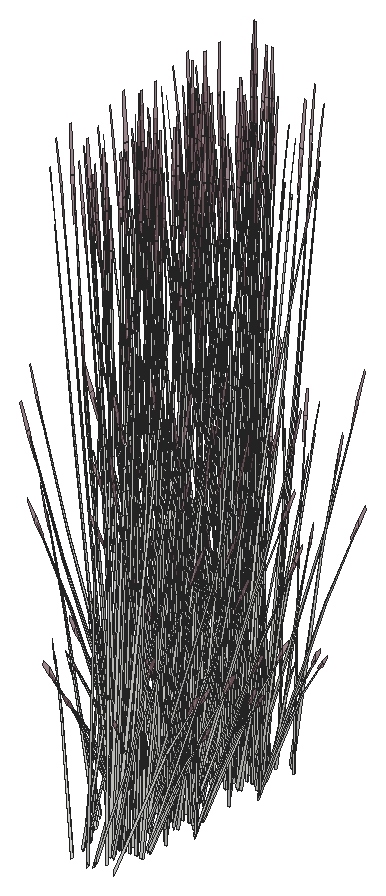
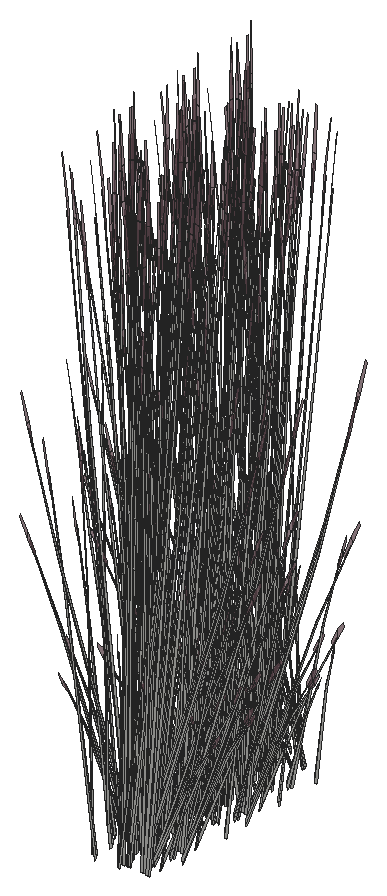
# SketchUp Ruby script. Lengths in inches.
U = 1.inch
M = Sketchup.active_model
def pt(a) = Geom::Point3d.new(a.map { |v| v * U })
def face(e, loops, mat)
  f = e.add_face(loops[0].map { |a| pt(a) })
  loops[1..].each { |l| e.add_face(l.map { |a| pt(a) }).erase! }
  f.material = f.back_material = mat if mat
  f
end
# faces: each face lists its corners as indices into pts; further lists are holes
def faces(e, pts, list, mat = nil) = list.each { |f| face(e, (f[0].is_a?(Array) ? f : [f]).map { |l| l.map { |i| pts[i] } }, mat) }
# xy, xz, yz: faces in a plane at the given z, y or x. An outline is a flat list of corners, or four numbers for a rectangle; further outlines are holes
def ring(l) = l.size == 4 ? [[l[0], l[1]], [l[2], l[1]], [l[2], l[3]], [l[0], l[3]]] : l.each_slice(2).to_a
def flat(e, list, mat, &to3) = list.each { |f| face(e, (f[0].is_a?(Array) ? f : [f]).map { |l| ring(l).map { |u, v| to3.(u, v) } }, mat) }
def xy(e, z, list, mat = nil) = flat(e, list, mat) { |x, y| [x, y, z] }
def xz(e, y, list, mat = nil) = flat(e, list, mat) { |x, z| [x, y, z] }
def yz(e, x, list, mat = nil) = flat(e, list, mat) { |y, z| [x, y, z] }
def lines(e, pts, list) = list.each { |a, b| e.add_line(pt(pts[a]), pt(pts[b])) }
# prism: a flat outline (further loops are holes) pulled along v
def prism(e, loops, v, mat = nil)
  f = face(e, loops, mat); d = Geom::Vector3d.new(v.map { |x| x * U })
  f.pushpull(f.normal.samedirection?(d) ? d.length : -d.length)
end
def box(e, o, s, mat = nil) = prism(e, [[o, [o[0] + s[0], o[1], o[2]], [o[0] + s[0], o[1] + s[1], o[2]], [o[0], o[1] + s[1], o[2]]]], [0, 0, s[2]], mat)
def at(x, y, z, deg = 0) = Geom::Transformation.translation(pt([x, y, z])) * Geom::Transformation.rotation(ORIGIN, Z_AXIS, deg.degrees)
def axes(o, x, y, z) = Geom::Transformation.new([*x, 0, *y, 0, *z, 0, *pt(o).to_a, 1])
def part(name) = M.definitions.add(name)
# library, detail: a bought-in or finely detailed component or shape, given as its bounding box
def library(name, o, s) = part(name).tap { |d| box(d.entities, o, s) }
def detail(e, o, s) = box(e.add_group.entities, o, s)
def put(e, d, t, mat = nil) = e.add_instance(d, t).tap { |i| i.material = mat if mat }
def group(e, t, mat = nil) = e.add_group.tap { |g| g.transformation = t; g.material = mat if mat }.entities
root = M.entities
M.materials.add("LightPink_Translucent").color = [144, 107, 117]
M.materials["LightPink_Translucent"].alpha = 0.75
c1 = part("blade")
p = [[2.15,0.21,22],[0,0.17,0],[0.09,0.45,0],[2.18,0.31,22],[2.29,0.31,22],[0.38,0.45,0],
  [2.48,0.24,33],[2.49,0.24,33],[2.48,0.22,33]]
faces(c1.entities,p,[[0,1,2,3],[4,5,2,3],[6,3,4,7],[8,0,3,6]])
c2 = part("seeds")
p = [[0.3,-0.1,1.38],[-0.01,-0.03,1.59],[-0.01,-0.03,0.03],[0.14,-0.07,-0.07],[0.29,-0.03,3],[0.15,0.01,3.11]]
faces(c2.entities,p,[[0,1,2,3],[1,0,4,5]],"LightPink_Translucent")
c3 = part("blade with seeds")
put(c3.entities,c1,at(0,0,0))
put(c3.entities,c2,axes([2.4,0.25,30.99],[1.5799,-0.05474,1.17369],[-0.12525,1.92788,0.29478],[-0.07173,-0.02425,1.56792]))
put(root,c3,axes([428.55,445.8,152.09],[0.44036,-0.12519,0.14904],[0.10874,0.46588,0.29641],[-0.03927,-0.06788,1.35512]))
put(root,c3,axes([429.46,444.04,152.25],[0.41376,-0.31314,-0.2458],[0.27514,0.44246,-0.42242],[0.10209,0.04493,1.34921]))
put(root,c3,axes([430.08,442.71,152],[0.25622,0.47263,0],[-0.42866,0.26357,-0.43598],[-0.09763,0.06003,1.38303]))
put(root,c3,axes([430.17,448.55,154.21],[0.01066,-0.43628,-0.60019],[0.44902,0.0293,0.07243],[0.04739,-0.18483,0.84903]))
put(root,c3,axes([430.48,442.87,151.26],[0.02986,-0.06809,1.48974],[0.37589,-0.20055,-0.22758],[0.11396,0.1038,0.25375]))
put(root,c3,axes([429.86,440.84,152.4],[-0.01119,-0.44408,1.19347],[0.50665,0.11511,0.50532],[-0.11983,0.243,1.12654]))
put(root,c3,axes([429.78,444.55,151.86],[0.45849,0,0],[0,0.4883,0],[0,0,1.50718]))
put(root,c3,axes([427.03,442.82,151.26],[0.05497,0.04712,1.48974],[0.09321,0.43661,-0.22758],[-0.12183,0.0931,0.25375]))
put(root,c3,axes([429,445.17,152.25],[-0.41376,0.31314,-0.2458],[-0.27514,-0.44246,-0.42242],[-0.10209,-0.04493,1.34921]))
put(root,c3,axes([429.91,443.41,152.09],[-0.44036,0.12519,0.14904],[-0.10874,-0.46588,0.29641],[0.03927,0.06788,1.35512]))
put(root,c3,axes([429.46,447.09,152.34],[0.05257,0.27504,0.97034],[-0.29163,-0.15233,0.71294],[0.03138,-0.14083,0.21373]))
put(root,c3,axes([430.46,442.99,152.25],[-0.26279,-0.01479,0.88755],[0.17355,-0.31417,0.49003],[0.10382,0.11162,0.6962]))
put(root,c3,axes([429.63,444.31,152.01],[-0.51796,-0.09937,0.41563],[0.10541,-0.56124,0.1631],[0.07569,0.05419,1.44303]))
put(root,c3,axes([429.21,445.69,151.86],[-0.13371,-0.40664,0],[0.38182,-0.1424,0],[0,0,1.30413]))
put(root,c3,axes([428.96,445.31,152.21],[-0.07906,0.42093,0.12232],[-0.38625,-0.07307,-0.3493],[-0.07029,-0.04322,1.07074]))
put(root,c3,axes([429.71,445.63,151.85],[0.43024,-0.16003,-0.16218],[0.15118,0.46099,0.00007],[0.04749,-0.01769,1.46908]))
put(root,c3,axes([429.86,445.83,152.09],[0.11838,-0.46875,0.14904],[0.43321,0.13265,0.29641],[-0.07483,0.00228,1.35512]))
put(root,c3,axes([429.77,444.76,151.87],[0.28606,0.30466,0],[-0.28606,0.30466,0],[0,0,1.42996]))
put(root,c3,axes([430.54,444.63,152.09],[-0.32198,-0.34356,0.14904],[0.32447,-0.33323,0.29641],[-0.03556,0.07016,1.35512]))
put(root,c3,axes([429.6,442.22,152.1875],[0.00723,-0.15635,1.20808],[0.34559,-0.17464,-0.25981],[0.10668,0.18713,0.51652]))
put(root,c3,axes([427.96,447.42,152.34],[0.21377,0.16416,0.97034],[-0.31132,0.09868,0.71294],[-0.06661,-0.12616,0.21373]))
put(root,c3,axes([431.83,444.95,152.34],[-0.2532,0.07787,0.97034],[0.11918,-0.32181,0.71294],[0.13432,0.02202,0.21373]))
put(root,c3,axes([428.47,448.29,154.21],[-0.34944,-0.22798,-0.60019],[0.24834,-0.39949,0.07243],[-0.1266,-0.13612,0.84903]))
put(root,c3,axes([429.12,445.875,151.86],[-0.41314,-0.21175,0],[0.19883,-0.43999,0],[0,0,1.37455]))
put(root,c3,axes([429.46,445.3125,152.08],[-0.40016,-0.37963,-0.21282],[0.33672,-0.42629,0.46574],[-0.10776,0.04441,1.42109]))
put(root,c3,axes([428.41,446.04,152.09],[0.38354,0.23583,0.41945],[-0.22925,0.42288,0],[-0.08735,-0.05371,1.33059]))
put(root,c3,axes([428.03,443.53,152.34],[-0.01061,-0.28045,0.97034],[0.26501,0.20003,0.71294],[-0.05212,0.13367,0.21373]))
put(root,c3,axes([429.76,444.41,152.3],[0.19883,-0.425,0.37796],[0.41314,0.20454,-0.1819],[0,0.09797,1.2135]))
put(root,c3,axes([428.73,442.86,151.26],[0.06632,-0.02567,1.48974],[0.39894,0.14126,-0.22758],[0.01167,0.15921,0.25375]))
put(root,c3,axes([429.68,444.65,151.9375],[0,0.54548,-0.04762],[-0.51243,0,0],[0,0.01714,1.5153]))
put(root,c3,axes([427.79,447.91,151.26],[-0.0397,0.06213,1.48974],[-0.40116,0.13396,-0.22758],[-0.09691,-0.12186,0.25375]))
put(root,c3,axes([428.1875,446.29,152],[-0.25622,0.47263,0],[-0.42866,-0.26357,-0.43598],[-0.09763,-0.06003,1.38303]))
put(root,c3,axes([430.8,444.64,152.09],[0,-0.47166,0.41945],[0.45849,0,0],[0,0.10742,1.33059]))
put(root,c3,axes([429.66,445,152.3],[0.44501,-0.02912,0.37796],[0.04024,0.48332,-0.1819],[-0.07967,0.04899,1.2135]))
put(root,c3,axes([429.93,444.5,152.21],[0.38182,-0.13755,0.12232],[0.13371,0.39278,-0.3493],[0,0.08644,1.07074]))
put(root,c3,axes([427.8125,442.92,152.38],[0.37228,-0.08352,0.05498],[0.08559,0.3365,-0.7291],[-0.0236,0.17034,0.65354]))
put(root,c3,axes([430.7,448.14,151.26],[-0.06134,-0.03716,1.48974],[-0.15755,-0.41512,-0.22758],[0.10629,-0.11265,0.25375]))
put(root,c3,axes([431.35,445.46,152.1875],[-0.0987,-0.116,1.20808],[0.12841,-0.38374,-0.25981],[0.19968,0.05198,0.51652]))
put(root,c3,axes([429.59,445.88,151.86],[0.41314,0.21175,0],[-0.19883,0.43999,0],[0,0,1.47801]))
put(root,c3,axes([430.7,449.3125,154.21],[0.21406,-0.37215,-0.60019],[0.37511,0.26448,0.07243],[0.12781,-0.13483,0.84903]))
put(root,c3,axes([428.38,448.23,152],[-0.25622,-0.47263,0],[0.42866,-0.26357,-0.43598],[0.09763,-0.06003,1.38303]))
put(root,c3,axes([429.75,446.35,151.85],[-0.25302,-0.47428,-0.04344],[0.42866,-0.26357,0.43598],[-0.10563,0.04516,1.38235]))
put(root,c3,axes([429.66,445.2,152.21],[0.30276,0.28338,0.12232],[-0.25254,0.31972,-0.3493],[-0.07029,0.04322,1.07074]))
put(root,c3,axes([428.95,447.66,151.8],[-0.28319,0.27058,-0.03288],[-0.25948,-0.29635,-0.1491],[-0.01827,-0.08397,0.4918]))
put(root,c3,axes([428.85,442.68,154.21],[0.19559,0.38351,-0.60019],[-0.40262,0.21373,0.07243],[0.04574,0.1853,0.84903]))
put(root,c3,axes([430.45,445.69,154.21],[0.40965,0.01136,-0.60019],[-0.02751,0.47821,0.07243],[0.17355,0.05047,0.84903]))
put(root,c3,axes([427.72,443.28,152.1875],[0.12932,-0.07441,1.20808],[0.31929,0.22435,-0.25981],[-0.09503,0.19413,0.51652]))
put(root,c3,axes([429.99,446.08,152.09],[0.38354,-0.23583,0.41945],[0.22925,0.42288,0],[-0.08735,0.05371,1.33059]))
put(root,c3,axes([429.44,445.71,151.9375],[0.17817,0.54185,-0.05079],[-0.50909,0.18987,0],[0.00622,0.01892,1.45452]))
put(root,c3,axes([426.88,445.46,152.1875],[0.14242,0.03872,1.20808],[0.09179,0.39548,-0.25981],[-0.19345,0.07403,0.51652]))
put(root,c3,axes([431.01,448.97,152.1875],[-0.1464,-0.01397,1.20808],[-0.14998,-0.37477,-0.25981],[0.17985,-0.10602,0.51652]))
put(root,c3,axes([431.12,444.72,152.01],[0.51243,0,0],[0,0.52715,-0.43598],[0,0.12006,1.38303]))
put(root,c3,axes([430.91,445,151.86],[-0.51218,-0.00377,-0.04204],[0,-0.52715,0.42192],[-0.0161,0.12,1.33776]))
put(root,c3,axes([429.8,444.54,152.25],[0.46151,0.22505,-0.2458],[-0.22222,0.475,-0.42242],[0.0145,0.11662,1.34921]))
put(root,c3,axes([431.18,448.28,152.34],[-0.1365,0.2401,0.97034],[-0.11733,-0.32258,0.71294],[0.11274,-0.08083,0.21373]))
put(root,c3,axes([426.58,446.29,152.34],[0.17079,-0.21377,0.97034],[0.06739,0.33841,0.71294],[-0.12342,0.0606,0.21373]))
put(root,c3,axes([429.57,445.1,152.25],[0.04775,0.53819,-0.2458],[-0.49736,0.03254,-0.42242],[-0.08758,0.07169,1.34921]))
put(root,c3,axes([428.89,449.53,152.25],[-0.04775,-0.53819,-0.2458],[0.49736,-0.03254,-0.42242],[0.08758,-0.07169,1.34921]))
put(root,c3,axes([427.54,448.15,151.8],[-0.11822,0.38513,-0.03288],[-0.36385,-0.11847,-0.1491],[-0.05524,-0.06299,0.4918]))
put(root,c3,axes([428.66,450.1,152.25],[-0.46151,-0.22505,-0.2458],[0.22222,-0.475,-0.42242],[-0.0145,-0.11662,1.34921]))
put(root,c3,axes([427.34,449.91,152],[-0.51243,0,0],[0,-0.52715,-0.43598],[0,-0.12006,1.38303]))
put(root,c3,axes([429.76,446.11,151.97],[0.51304,0.1533,0.25983],[-0.12835,0.54797,-0.30828],[-0.08491,0.06858,1.39295]))
put(root,c3,axes([427.43,448.97,152.1875],[0.08001,0.13132,1.20808],[-0.18437,0.35694,-0.25981],[-0.18931,-0.08532,0.51652]))
put(root,c3,axes([427.76,448.85,154.21],[-0.40965,-0.01136,-0.60019],[0.02751,-0.47821,0.07243],[-0.17355,-0.05047,0.84903]))
put(root,c3,axes([430.42,446.0625,152.34],[-0.23074,-0.13562,0.97034],[0.29794,-0.1378,0.71294],[0.08036,0.11673,0.21373]))
put(root,c3,axes([427.74,449.77,151.97],[-0.38118,0.39654,0.25983],[-0.38142,-0.39237,-0.30828],[-0.01331,-0.11261,1.39295]))
put(root,c3,axes([430.08,446.41,152],[0.25622,0.47263,0],[-0.42866,0.26357,-0.43598],[-0.09763,0.06003,1.38303]))
put(root,c3,axes([430.48,446.5625,151.26],[0.02986,-0.06809,1.48974],[0.37589,-0.20055,-0.22758],[0.11396,0.1038,0.25375]))
put(root,c3,axes([429.86,444.53,152.4],[-0.01119,-0.44408,1.19347],[0.50665,0.11511,0.50532],[-0.11983,0.243,1.12654]))
put(root,c3,axes([427.03,446.51,151.26],[0.05497,0.04712,1.48974],[0.09321,0.43661,-0.22758],[-0.12183,0.0931,0.25375]))
put(root,c3,axes([428.95,449.95,152.06],[0.46174,0.2286,0.2033],[-0.22222,0.475,0.42242],[0,-0.1095,1.35626]))
put(root,c3,axes([428.77,450.6,152.06],[0.10862,-0.55889,-0.19793],[0.515,0.09742,0.43313],[-0.08999,-0.07718,1.32161]))
put(root,c3,axes([426.95,449.36,152.34],[0.26163,-0.03375,0.97034],[-0.16596,0.29737,0.71294],[-0.12929,-0.04461,0.21373]))
put(root,c3,axes([430.46,446.68,152.25],[-0.26279,-0.01479,0.88755],[0.17355,-0.31417,0.49003],[0.10382,0.11162,0.6962]))
put(root,c3,axes([428.8,449.64,152.3],[-0.44501,0.02912,0.37796],[-0.04024,-0.48332,-0.1819],[0.07967,-0.04899,1.2135]))
put(root,c3,axes([427.65,449.99,152.09],[0,0.47166,0.41945],[-0.45849,0,0],[0,-0.10742,1.33059]))
put(root,c3,axes([430.27,448.35,152.01],[0.25622,-0.47263,0],[0.42866,0.26357,-0.43598],[0.09763,0.06003,1.38303]))
put(root,c3,axes([428.79,449.81,151.99],[0.17817,0.52741,0.38653],[-0.50909,0.1834,0.15168],[0.00622,-0.09691,1.34202]))
put(root,c3,axes([431.28,450.21,151.67],[-0.26394,0.0566,1.1961],[-0.04201,-0.45055,0.06846],[0.18486,-0.06819,0.68062]))
put(root,c3,axes([431.76,449.82,151.91],[-0.25407,-0.3016,-0.05481],[0.27826,-0.27635,-0.2485],[0.07884,-0.01946,0.81966]))
put(root,c3,axes([428.7,450.23,152.3],[-0.19883,0.425,0.37796],[-0.41314,-0.20454,-0.1819],[0,-0.09797,1.2135]))
put(root,c3,axes([429.6,445.92,152.1875],[0.00723,-0.15635,1.20808],[0.34559,-0.17464,-0.25981],[0.10668,0.18713,0.51652]))
put(root,c3,axes([429.43,449.85,151.86],[0,-0.54574,0],[0.51243,0,0],[0,0,1.51605]))
put(root,c3,axes([430.05,448.59,152.09],[-0.38354,-0.23583,0.41945],[0.22925,-0.42288,0],[0.08735,0.05371,1.33059]))
put(root,c3,axes([430.8,450.25,154.21],[0.3601,-0.20831,-0.60019],[0.20068,0.4288,0.07243],[0.17399,-0.04871,0.84903]))
put(root,c3,axes([428.03,447.22,152.34],[-0.01061,-0.28045,0.97034],[0.26501,0.20003,0.71294],[-0.05212,0.13367,0.21373]))
put(root,c3,axes([429.18,449.51,151.99],[-0.33979,0.42804,0.38653],[-0.40368,-0.37784,0.15168],[0.08192,-0.04272,1.34202]))
put(root,c3,axes([429.56,450.28,151.94],[-0.38118,-0.40596,-0.0518],[0.38142,-0.40621,0],[-0.01331,-0.01418,1.48322]))
put(root,c3,axes([428.59,448.81,152.09],[-0.11838,0.46875,0.14904],[-0.43321,-0.13265,0.29641],[0.07483,-0.00228,1.35512]))
put(root,c3,axes([428.73,446.55,151.26],[0.06632,-0.02567,1.48974],[0.39894,0.14126,-0.22758],[0.01167,0.15921,0.25375]))
put(root,c3,axes([428.42,449.18,151.35],[-0.40337,0.18883,1.08919],[-0.12839,-0.54182,0.42321],[0.24769,0.00901,1.23883]))
put(root,c3,axes([429.5,449.33,152.21],[0.07906,-0.42093,0.12232],[0.38625,0.07307,-0.3493],[0.07029,0.04322,1.07074]))
put(root,c3,axes([428.83,450.33,151.99],[0.51796,0.09937,0.38653],[-0.10541,0.56124,0.15168],[-0.07569,-0.05419,1.34202]))
put(root,c3,axes([431.57,449.92,151.26],[-0.02142,-0.07161,1.48974],[0.14855,-0.41887,-0.22758],[0.14984,-0.00603,0.25375]))
put(root,c3,axes([427.8125,446.61,152.38],[0.37228,-0.08352,0.05498],[0.08559,0.3365,-0.7291],[-0.0236,0.17034,0.65354]))
put(root,c3,axes([427.14,449.85,151.26],[0.01039,0.07433,1.48974],[-0.20952,0.38819,-0.22758],[-0.14882,-0.01957,0.25375]))
put(root,c3,axes([429.33,449.4375,152.3],[-0.24618,-0.39589,0.37796],[0.37289,-0.27878,-0.1819],[0.07967,0.04899,1.2135]))
put(root,c3,axes([428.55,451.22,152.09],[0.44036,-0.12519,0.14904],[0.10874,0.46588,0.29641],[-0.03927,-0.06788,1.35512]))
put(root,c3,axes([429.46,449.46,152.25],[0.41376,-0.31314,-0.2458],[0.27514,0.44246,-0.42242],[0.10209,0.04493,1.34921]))
put(root,c3,axes([429.78,449.98,151.86],[0.45849,0,0],[0,0.4883,0],[0,0,1.50718]))
put(root,c3,axes([429,450.59,152.25],[-0.41376,0.31314,-0.2458],[-0.27514,-0.44246,-0.42242],[-0.10209,-0.04493,1.34921]))
put(root,c3,axes([429.91,448.83,152.09],[-0.44036,0.12519,0.14904],[-0.10874,-0.46588,0.29641],[0.03927,0.06788,1.35512]))
put(root,c3,axes([428.85,446.37,154.21],[0.19559,0.38351,-0.60019],[-0.40262,0.21373,0.07243],[0.04574,0.1853,0.84903]))
put(root,c3,axes([427.72,446.97,152.1875],[0.12932,-0.07441,1.20808],[0.31929,0.22435,-0.25981],[-0.09503,0.19413,0.51652]))
put(root,c3,axes([429.63,449.73,152.01],[-0.51796,-0.09937,0.41563],[0.10541,-0.56124,0.1631],[0.07569,0.05419,1.44303]))
put(root,c3,axes([429.21,451.11,151.86],[-0.13371,-0.40664,0],[0.38182,-0.1424,0],[0,0,1.30413]))
put(root,c3,axes([428.96,450.73,152.21],[-0.07906,0.42093,0.12232],[-0.38625,-0.07307,-0.3493],[-0.07029,-0.04322,1.07074]))
put(root,c3,axes([429.71,451.06,151.85],[0.43024,-0.16003,-0.16218],[0.15118,0.46099,0.00007],[0.04749,-0.01769,1.46908]))
put(root,c3,axes([429.86,451.25,152.09],[0.11838,-0.46875,0.14904],[0.43321,0.13265,0.29641],[-0.07483,0.00228,1.35512]))
put(root,c3,axes([429.88,454.33,152.1875],[-0.11649,0.09547,1.20808],[-0.34886,-0.1671,-0.25981],[0.06467,-0.20781,0.51652]))
put(root,c3,axes([429.77,450.1875,151.87],[0.28606,0.30466,0],[-0.28606,0.30466,0],[0,0,1.42996]))
put(root,c3,axes([429.35,454.66,154.21],[-0.19559,-0.38351,-0.60019],[0.40262,-0.21373,0.07243],[-0.04574,-0.1853,0.84903]))
put(root,c3,axes([430.54,450.05,152.09],[-0.32198,-0.34356,0.14904],[0.32447,-0.33323,0.29641],[-0.03556,0.07016,1.35512]))
put(root,c3,axes([428.08,454.15,152.1875],[-0.02482,0.15429,1.20808],[-0.36278,0.12916,-0.25981],[-0.0848,-0.19943,0.51652]))
put(root,c3,axes([431.83,450.37,152.34],[-0.2532,0.07787,0.97034],[0.11918,-0.32181,0.71294],[0.13432,0.02202,0.21373]))
put(root,c3,axes([429.12,451.3,151.86],[-0.41314,-0.21175,0],[0.19883,-0.43999,0],[0,0,1.37455]))
put(root,c3,axes([429.46,450.73,152.08],[-0.40016,-0.37963,-0.21282],[0.33672,-0.42629,0.46574],[-0.10776,0.04441,1.42109]))
put(root,c3,axes([429.02,453.81,151.26],[-0.06874,0.01699,1.48974],[-0.38012,-0.19128,-0.22758],[0.00638,-0.15955,0.25375]))
put(root,c3,axes([428.41,451.46,152.09],[0.38354,0.23583,0.41945],[-0.22925,0.42288,0],[-0.08735,-0.05371,1.33059]))
put(root,c3,axes([429.76,449.83,152.3],[0.19883,-0.425,0.37796],[0.41314,0.20454,-0.1819],[0,0.09797,1.2135]))
put(root,c3,axes([430.17,455.04,154.21],[0.01066,-0.43628,-0.60019],[0.44902,0.0293,0.07243],[0.04739,-0.18483,0.84903]))
put(root,c3,axes([429.68,450.07,151.9375],[0,0.54548,-0.04762],[-0.51243,0,0],[0,0.01714,1.5153]))
put(root,c3,axes([428.1875,451.71,152],[-0.25622,0.47263,0],[-0.42866,-0.26357,-0.43598],[-0.09763,-0.06003,1.38303]))
put(root,c3,axes([430.8,450.07,152.09],[0,-0.47166,0.41945],[0.45849,0,0],[0,0.10742,1.33059]))
put(root,c3,axes([429.66,450.42,152.3],[0.44501,-0.02912,0.37796],[0.04024,0.48332,-0.1819],[-0.07967,0.04899,1.2135]))
put(root,c3,axes([429.93,449.93,152.21],[0.38182,-0.13755,0.12232],[0.13371,0.39278,-0.3493],[0,0.08644,1.07074]))
put(root,c3,axes([429.46,453.57,152.34],[0.05257,0.27504,0.97034],[-0.29163,-0.15233,0.71294],[0.03138,-0.14083,0.21373]))
put(root,c3,axes([431.35,450.88,152.1875],[-0.0987,-0.116,1.20808],[0.12841,-0.38374,-0.25981],[0.19968,0.05198,0.51652]))
put(root,c3,axes([429.59,451.31,151.86],[0.41314,0.21175,0],[-0.19883,0.43999,0],[0,0,1.47801]))
put(root,c3,axes([429.75,451.77,151.85],[-0.25302,-0.47428,-0.04344],[0.42866,-0.26357,0.43598],[-0.10563,0.04516,1.38235]))
put(root,c3,axes([427.96,453.9,152.34],[0.21377,0.16416,0.97034],[-0.31132,0.09868,0.71294],[-0.06661,-0.12616,0.21373]))
put(root,c3,axes([429.66,450.63,152.21],[0.30276,0.28338,0.12232],[-0.25254,0.31972,-0.3493],[-0.07029,0.04322,1.07074]))
put(root,c3,axes([428.47,454.77,154.21],[-0.34944,-0.22798,-0.60019],[0.24834,-0.39949,0.07243],[-0.1266,-0.13612,0.84903]))
put(root,c3,axes([430.45,451.12,154.21],[0.40965,0.01136,-0.60019],[-0.02751,0.47821,0.07243],[0.17355,0.05047,0.84903]))
put(root,c3,axes([429.99,451.5,152.09],[0.38354,-0.23583,0.41945],[0.22925,0.42288,0],[-0.08735,0.05371,1.33059]))
put(root,c3,axes([429.44,451.13,151.9375],[0.17817,0.54185,-0.05079],[-0.50909,0.18987,0],[0.00622,0.01892,1.45452]))
put(root,c3,axes([427.79,454.39,151.26],[-0.0397,0.06213,1.48974],[-0.40116,0.13396,-0.22758],[-0.09691,-0.12186,0.25375]))
put(root,c3,axes([426.88,450.88,152.1875],[0.14242,0.03872,1.20808],[0.09179,0.39548,-0.25981],[-0.19345,0.07403,0.51652]))
put(root,c3,axes([431.12,450.15,152.01],[0.51243,0,0],[0,0.52715,-0.43598],[0,0.12006,1.38303]))
put(root,c3,axes([430.7,454.62,151.26],[-0.06134,-0.03716,1.48974],[-0.15755,-0.41512,-0.22758],[0.10629,-0.11265,0.25375]))
put(root,c3,axes([430.91,450.42,151.86],[-0.51218,-0.00377,-0.04204],[0,-0.52715,0.42192],[-0.0161,0.12,1.33776]))
put(root,c3,axes([429.8,449.96,152.25],[0.46151,0.22505,-0.2458],[-0.22222,0.475,-0.42242],[0.0145,0.11662,1.34921]))
put(root,c3,axes([426.58,451.71,152.34],[0.17079,-0.21377,0.97034],[0.06739,0.33841,0.71294],[-0.12342,0.0606,0.21373]))
put(root,c3,axes([429.57,450.52,152.25],[0.04775,0.53819,-0.2458],[-0.49736,0.03254,-0.42242],[-0.08758,0.07169,1.34921]))
put(root,c3,axes([430.7,455.79,154.21],[0.21406,-0.37215,-0.60019],[0.37511,0.26448,0.07243],[0.12781,-0.13483,0.84903]))
put(root,c3,axes([428.38,454.71,152],[-0.25622,-0.47263,0],[0.42866,-0.26357,-0.43598],[0.09763,-0.06003,1.38303]))
put(root,c3,axes([428.95,454.14,151.8],[-0.28319,0.27058,-0.03288],[-0.25948,-0.29635,-0.1491],[-0.01827,-0.08397,0.4918]))
put(root,c3,axes([429.76,451.53,151.97],[0.51304,0.1533,0.25983],[-0.12835,0.54797,-0.30828],[-0.08491,0.06858,1.39295]))
put(root,c3,axes([430.42,451.48,152.34],[-0.23074,-0.13562,0.97034],[0.29794,-0.1378,0.71294],[0.08036,0.11673,0.21373]))
put(root,c3,axes([431.01,455.45,152.1875],[-0.1464,-0.01397,1.20808],[-0.14998,-0.37477,-0.25981],[0.17985,-0.10602,0.51652]))
put(root,c3,axes([431.18,454.76,152.34],[-0.1365,0.2401,0.97034],[-0.11733,-0.32258,0.71294],[0.11274,-0.08083,0.21373]))
put(root,c3,axes([430.08,451.83,152],[0.25622,0.47263,0],[-0.42866,0.26357,-0.43598],[-0.09763,0.06003,1.38303]))
put(root,c3,axes([430.48,451.99,151.26],[0.02986,-0.06809,1.48974],[0.37589,-0.20055,-0.22758],[0.11396,0.1038,0.25375]))
put(root,c3,axes([429.86,449.96,152.4],[-0.01119,-0.44408,1.19347],[0.50665,0.11511,0.50532],[-0.11983,0.243,1.12654]))
put(root,c3,axes([427.03,451.93,151.26],[0.05497,0.04712,1.48974],[0.09321,0.43661,-0.22758],[-0.12183,0.0931,0.25375]))
put(root,c3,axes([428.89,456.02,152.25],[-0.04775,-0.53819,-0.2458],[0.49736,-0.03254,-0.42242],[0.08758,-0.07169,1.34921]))
put(root,c3,axes([427.54,454.63,151.8],[-0.11822,0.38513,-0.03288],[-0.36385,-0.11847,-0.1491],[-0.05524,-0.06299,0.4918]))
put(root,c3,axes([430.46,452.1,152.25],[-0.26279,-0.01479,0.88755],[0.17355,-0.31417,0.49003],[0.10382,0.11162,0.6962]))
put(root,c3,axes([428.66,456.58,152.25],[-0.46151,-0.22505,-0.2458],[0.22222,-0.475,-0.42242],[-0.0145,-0.11662,1.34921]))
put(root,c3,axes([427.34,456.39,152],[-0.51243,0,0],[0,-0.52715,-0.43598],[0,-0.12006,1.38303]))
put(root,c3,axes([427.43,455.45,152.1875],[0.08001,0.13132,1.20808],[-0.18437,0.35694,-0.25981],[-0.18931,-0.08532,0.51652]))
put(root,c3,axes([429.88,457.875,152.1875],[-0.11649,0.09547,1.20808],[-0.34886,-0.1671,-0.25981],[0.06467,-0.20781,0.51652]))
put(root,c3,axes([429.35,458.21,154.21],[-0.19559,-0.38351,-0.60019],[0.40262,-0.21373,0.07243],[-0.04574,-0.1853,0.84903]))
put(root,c3,axes([427.76,455.33,154.21],[-0.40965,-0.01136,-0.60019],[0.02751,-0.47821,0.07243],[-0.17355,-0.05047,0.84903]))
put(root,c3,axes([428.08,457.69,152.1875],[-0.02482,0.15429,1.20808],[-0.36278,0.12916,-0.25981],[-0.0848,-0.19943,0.51652]))
put(root,c3,axes([429.02,457.36,151.26],[-0.06874,0.01699,1.48974],[-0.38012,-0.19128,-0.22758],[0.00638,-0.15955,0.25375]))
put(root,c3,axes([429.6,451.34,152.1875],[0.00723,-0.15635,1.20808],[0.34559,-0.17464,-0.25981],[0.10668,0.18713,0.51652]))
put(root,c3,axes([430.17,458.58,154.21],[0.01066,-0.43628,-0.60019],[0.44902,0.0293,0.07243],[0.04739,-0.18483,0.84903]))
put(root,c3,axes([428.03,452.64,152.34],[-0.01061,-0.28045,0.97034],[0.26501,0.20003,0.71294],[-0.05212,0.13367,0.21373]))
put(root,c3,axes([427.74,456.25,151.97],[-0.38118,0.39654,0.25983],[-0.38142,-0.39237,-0.30828],[-0.01331,-0.11261,1.39295]))
put(root,c3,axes([428.73,451.97,151.26],[0.06632,-0.02567,1.48974],[0.39894,0.14126,-0.22758],[0.01167,0.15921,0.25375]))
put(root,c3,axes([428.95,456.4375,152.06],[0.46174,0.2286,0.2033],[-0.22222,0.475,0.42242],[0,-0.1095,1.35626]))
put(root,c3,axes([428.77,457.08,152.06],[0.10862,-0.55889,-0.19793],[0.515,0.09742,0.43313],[-0.08999,-0.07718,1.32161]))
put(root,c3,axes([429.46,457.12,152.34],[0.05257,0.27504,0.97034],[-0.29163,-0.15233,0.71294],[0.03138,-0.14083,0.21373]))
put(root,c3,axes([426.95,455.84,152.34],[0.26163,-0.03375,0.97034],[-0.16596,0.29737,0.71294],[-0.12929,-0.04461,0.21373]))
put(root,c3,axes([427.8125,452.04,152.38],[0.37228,-0.08352,0.05498],[0.08559,0.3365,-0.7291],[-0.0236,0.17034,0.65354]))
put(root,c3,axes([428.8,456.12,152.3],[-0.44501,0.02912,0.37796],[-0.04024,-0.48332,-0.1819],[0.07967,-0.04899,1.2135]))
put(root,c3,axes([427.65,456.47,152.09],[0,0.47166,0.41945],[-0.45849,0,0],[0,-0.10742,1.33059]))
put(root,c3,axes([430.27,454.83,152.01],[0.25622,-0.47263,0],[0.42866,0.26357,-0.43598],[0.09763,0.06003,1.38303]))
put(root,c3,axes([428.79,456.29,151.99],[0.17817,0.52741,0.38653],[-0.50909,0.1834,0.15168],[0.00622,-0.09691,1.34202]))
put(root,c3,axes([427.96,457.45,152.34],[0.21377,0.16416,0.97034],[-0.31132,0.09868,0.71294],[-0.06661,-0.12616,0.21373]))
put(root,c3,axes([428.47,458.32,154.21],[-0.34944,-0.22798,-0.60019],[0.24834,-0.39949,0.07243],[-0.1266,-0.13612,0.84903]))
put(root,c3,axes([431.28,456.7,151.67],[-0.26394,0.0566,1.1961],[-0.04201,-0.45055,0.06846],[0.18486,-0.06819,0.68062]))
put(root,c3,axes([431.76,456.3,151.91],[-0.25407,-0.3016,-0.05481],[0.27826,-0.27635,-0.2485],[0.07884,-0.01946,0.81966]))
put(root,c3,axes([428.7,456.71,152.3],[-0.19883,0.425,0.37796],[-0.41314,-0.20454,-0.1819],[0,-0.09797,1.2135]))
put(root,c3,axes([429.43,456.34,151.86],[0,-0.54574,0],[0.51243,0,0],[0,0,1.51605]))
put(root,c3,axes([430.05,455.08,152.09],[-0.38354,-0.23583,0.41945],[0.22925,-0.42288,0],[0.08735,0.05371,1.33059]))
put(root,c3,axes([430.8,456.73,154.21],[0.3601,-0.20831,-0.60019],[0.20068,0.4288,0.07243],[0.17399,-0.04871,0.84903]))
put(root,c3,axes([428.85,451.79,154.21],[0.19559,0.38351,-0.60019],[-0.40262,0.21373,0.07243],[0.04574,0.1853,0.84903]))
put(root,c3,axes([429.18,455.99,151.99],[-0.33979,0.42804,0.38653],[-0.40368,-0.37784,0.15168],[0.08192,-0.04272,1.34202]))
put(root,c3,axes([429.56,456.76,151.94],[-0.38118,-0.40596,-0.0518],[0.38142,-0.40621,0],[-0.01331,-0.01418,1.48322]))
put(root,c3,axes([427.72,452.39,152.1875],[0.12932,-0.07441,1.20808],[0.31929,0.22435,-0.25981],[-0.09503,0.19413,0.51652]))
put(root,c3,axes([427.79,457.94,151.26],[-0.0397,0.06213,1.48974],[-0.40116,0.13396,-0.22758],[-0.09691,-0.12186,0.25375]))
put(root,c3,axes([428.59,455.29,152.09],[-0.11838,0.46875,0.14904],[-0.43321,-0.13265,0.29641],[0.07483,-0.00228,1.35512]))
put(root,c3,axes([430.7,458.17,151.26],[-0.06134,-0.03716,1.48974],[-0.15755,-0.41512,-0.22758],[0.10629,-0.11265,0.25375]))
put(root,c3,axes([428.42,455.67,151.35],[-0.40337,0.18883,1.08919],[-0.12839,-0.54182,0.42321],[0.24769,0.00901,1.23883]))
put(root,c3,axes([429.5,455.81,152.21],[0.07906,-0.42093,0.12232],[0.38625,0.07307,-0.3493],[0.07029,0.04322,1.07074]))
put(root,c3,axes([428.83,456.81,151.99],[0.51796,0.09937,0.38653],[-0.10541,0.56124,0.15168],[-0.07569,-0.05419,1.34202]))
put(root,c3,axes([431.57,456.4,151.26],[-0.02142,-0.07161,1.48974],[0.14855,-0.41887,-0.22758],[0.14984,-0.00603,0.25375]))
put(root,c3,axes([427.14,456.33,151.26],[0.01039,0.07433,1.48974],[-0.20952,0.38819,-0.22758],[-0.14882,-0.01957,0.25375]))
put(root,c3,axes([429.33,455.92,152.3],[-0.24618,-0.39589,0.37796],[0.37289,-0.27878,-0.1819],[0.07967,0.04899,1.2135]))
put(root,c3,axes([428.55,457.71,152.09],[0.44036,-0.12519,0.14904],[0.10874,0.46588,0.29641],[-0.03927,-0.06788,1.35512]))
put(root,c3,axes([429.46,455.95,152.25],[0.41376,-0.31314,-0.2458],[0.27514,0.44246,-0.42242],[0.10209,0.04493,1.34921]))
put(root,c3,axes([430.7,459.34,154.21],[0.21406,-0.37215,-0.60019],[0.37511,0.26448,0.07243],[0.12781,-0.13483,0.84903]))
put(root,c3,axes([428.38,458.26,152],[-0.25622,-0.47263,0],[0.42866,-0.26357,-0.43598],[0.09763,-0.06003,1.38303]))
put(root,c3,axes([428.95,457.6875,151.8],[-0.28319,0.27058,-0.03288],[-0.25948,-0.29635,-0.1491],[-0.01827,-0.08397,0.4918]))
put(root,c3,axes([429.78,456.46,151.86],[0.45849,0,0],[0,0.4883,0],[0,0,1.50718]))
put(root,c3,axes([429,457.07,152.25],[-0.41376,0.31314,-0.2458],[-0.27514,-0.44246,-0.42242],[-0.10209,-0.04493,1.34921]))
put(root,c3,axes([429.91,455.3125,152.09],[-0.44036,0.12519,0.14904],[-0.10874,-0.46588,0.29641],[0.03927,0.06788,1.35512]))
put(root,c3,axes([429.63,456.21,152.01],[-0.51796,-0.09937,0.41563],[0.10541,-0.56124,0.1631],[0.07569,0.05419,1.44303]))
put(root,c3,axes([429.21,457.6,151.86],[-0.13371,-0.40664,0],[0.38182,-0.1424,0],[0,0,1.30413]))
put(root,c3,axes([431.01,459,152.1875],[-0.1464,-0.01397,1.20808],[-0.14998,-0.37477,-0.25981],[0.17985,-0.10602,0.51652]))
put(root,c3,axes([428.96,457.21,152.21],[-0.07906,0.42093,0.12232],[-0.38625,-0.07307,-0.3493],[-0.07029,-0.04322,1.07074]))
put(root,c3,axes([429.71,457.54,151.85],[0.43024,-0.16003,-0.16218],[0.15118,0.46099,0.00007],[0.04749,-0.01769,1.46908]))
put(root,c3,axes([429.86,457.73,152.09],[0.11838,-0.46875,0.14904],[0.43321,0.13265,0.29641],[-0.07483,0.00228,1.35512]))
put(root,c3,axes([431.18,458.31,152.34],[-0.1365,0.2401,0.97034],[-0.11733,-0.32258,0.71294],[0.11274,-0.08083,0.21373]))
put(root,c3,axes([429.77,456.67,151.87],[0.28606,0.30466,0],[-0.28606,0.30466,0],[0,0,1.42996]))
put(root,c3,axes([430.54,456.54,152.09],[-0.32198,-0.34356,0.14904],[0.32447,-0.33323,0.29641],[-0.03556,0.07016,1.35512]))
put(root,c3,axes([431.83,456.85,152.34],[-0.2532,0.07787,0.97034],[0.11918,-0.32181,0.71294],[0.13432,0.02202,0.21373]))
put(root,c3,axes([429.12,457.78,151.86],[-0.41314,-0.21175,0],[0.19883,-0.43999,0],[0,0,1.37455]))
put(root,c3,axes([429.46,457.22,152.08],[-0.40016,-0.37963,-0.21282],[0.33672,-0.42629,0.46574],[-0.10776,0.04441,1.42109]))
put(root,c3,axes([428.41,457.94,152.09],[0.38354,0.23583,0.41945],[-0.22925,0.42288,0],[-0.08735,-0.05371,1.33059]))
put(root,c3,axes([428.89,459.5625,152.25],[-0.04775,-0.53819,-0.2458],[0.49736,-0.03254,-0.42242],[0.08758,-0.07169,1.34921]))
put(root,c3,axes([429.76,456.3125,152.3],[0.19883,-0.425,0.37796],[0.41314,0.20454,-0.1819],[0,0.09797,1.2135]))
put(root,c3,axes([427.54,458.18,151.8],[-0.11822,0.38513,-0.03288],[-0.36385,-0.11847,-0.1491],[-0.05524,-0.06299,0.4918]))
put(root,c3,axes([428.66,460.125,152.25],[-0.46151,-0.22505,-0.2458],[0.22222,-0.475,-0.42242],[-0.0145,-0.11662,1.34921]))
put(root,c3,axes([429.68,456.56,151.9375],[0,0.54548,-0.04762],[-0.51243,0,0],[0,0.01714,1.5153]))
put(root,c3,axes([427.34,459.9375,152],[-0.51243,0,0],[0,-0.52715,-0.43598],[0,-0.12006,1.38303]))
put(root,c3,axes([427.43,459,152.1875],[0.08001,0.13132,1.20808],[-0.18437,0.35694,-0.25981],[-0.18931,-0.08532,0.51652]))
put(root,c3,axes([428.1875,458.19,152],[-0.25622,0.47263,0],[-0.42866,-0.26357,-0.43598],[-0.09763,-0.06003,1.38303]))
put(root,c3,axes([430.8,456.55,152.09],[0,-0.47166,0.41945],[0.45849,0,0],[0,0.10742,1.33059]))
put(root,c3,axes([429.66,456.9,152.3],[0.44501,-0.02912,0.37796],[0.04024,0.48332,-0.1819],[-0.07967,0.04899,1.2135]))
put(root,c3,axes([427.76,458.88,154.21],[-0.40965,-0.01136,-0.60019],[0.02751,-0.47821,0.07243],[-0.17355,-0.05047,0.84903]))
put(root,c3,axes([429.93,456.41,152.21],[0.38182,-0.13755,0.12232],[0.13371,0.39278,-0.3493],[0,0.08644,1.07074]))
put(root,c3,axes([431.35,457.37,152.1875],[-0.0987,-0.116,1.20808],[0.12841,-0.38374,-0.25981],[0.19968,0.05198,0.51652]))
put(root,c3,axes([429.59,457.79,151.86],[0.41314,0.21175,0],[-0.19883,0.43999,0],[0,0,1.47801]))
put(root,c3,axes([427.74,459.8,151.97],[-0.38118,0.39654,0.25983],[-0.38142,-0.39237,-0.30828],[-0.01331,-0.11261,1.39295]))
put(root,c3,axes([429.75,458.26,151.85],[-0.25302,-0.47428,-0.04344],[0.42866,-0.26357,0.43598],[-0.10563,0.04516,1.38235]))
put(root,c3,axes([429.66,457.11,152.21],[0.30276,0.28338,0.12232],[-0.25254,0.31972,-0.3493],[-0.07029,0.04322,1.07074]))
put(root,c3,axes([428.95,459.98,152.06],[0.46174,0.2286,0.2033],[-0.22222,0.475,0.42242],[0,-0.1095,1.35626]))
put(root,c3,axes([428.77,460.625,152.06],[0.10862,-0.55889,-0.19793],[0.515,0.09742,0.43313],[-0.08999,-0.07718,1.32161]))
put(root,c3,axes([426.95,459.39,152.34],[0.26163,-0.03375,0.97034],[-0.16596,0.29737,0.71294],[-0.12929,-0.04461,0.21373]))
put(root,c3,axes([430.45,457.6,154.21],[0.40965,0.01136,-0.60019],[-0.02751,0.47821,0.07243],[0.17355,0.05047,0.84903]))
put(root,c3,axes([429.99,457.98,152.09],[0.38354,-0.23583,0.41945],[0.22925,0.42288,0],[-0.08735,0.05371,1.33059]))
put(root,c3,axes([428.8,459.67,152.3],[-0.44501,0.02912,0.37796],[-0.04024,-0.48332,-0.1819],[0.07967,-0.04899,1.2135]))
put(root,c3,axes([427.65,460.02,152.09],[0,0.47166,0.41945],[-0.45849,0,0],[0,-0.10742,1.33059]))
put(root,c3,axes([429.44,457.61,151.9375],[0.17817,0.54185,-0.05079],[-0.50909,0.18987,0],[0.00622,0.01892,1.45452]))
put(root,c3,axes([430.27,458.375,152.01],[0.25622,-0.47263,0],[0.42866,0.26357,-0.43598],[0.09763,0.06003,1.38303]))
put(root,c3,axes([426.88,457.36,152.1875],[0.14242,0.03872,1.20808],[0.09179,0.39548,-0.25981],[-0.19345,0.07403,0.51652]))
put(root,c3,axes([428.79,459.84,151.99],[0.17817,0.52741,0.38653],[-0.50909,0.1834,0.15168],[0.00622,-0.09691,1.34202]))
put(root,c3,axes([431.12,456.63,152.01],[0.51243,0,0],[0,0.52715,-0.43598],[0,0.12006,1.38303]))
put(root,c3,axes([430.91,456.9,151.86],[-0.51218,-0.00377,-0.04204],[0,-0.52715,0.42192],[-0.0161,0.12,1.33776]))
put(root,c3,axes([429.8,456.44,152.25],[0.46151,0.22505,-0.2458],[-0.22222,0.475,-0.42242],[0.0145,0.11662,1.34921]))
put(root,c3,axes([431.28,460.24,151.67],[-0.26394,0.0566,1.1961],[-0.04201,-0.45055,0.06846],[0.18486,-0.06819,0.68062]))
put(root,c3,axes([431.76,459.84,151.91],[-0.25407,-0.3016,-0.05481],[0.27826,-0.27635,-0.2485],[0.07884,-0.01946,0.81966]))
put(root,c3,axes([426.58,458.19,152.34],[0.17079,-0.21377,0.97034],[0.06739,0.33841,0.71294],[-0.12342,0.0606,0.21373]))
put(root,c3,axes([428.7,460.26,152.3],[-0.19883,0.425,0.37796],[-0.41314,-0.20454,-0.1819],[0,-0.09797,1.2135]))
put(root,c3,axes([429.57,457.01,152.25],[0.04775,0.53819,-0.2458],[-0.49736,0.03254,-0.42242],[-0.08758,0.07169,1.34921]))
put(root,c3,axes([429.43,459.88,151.86],[0,-0.54574,0],[0.51243,0,0],[0,0,1.51605]))
